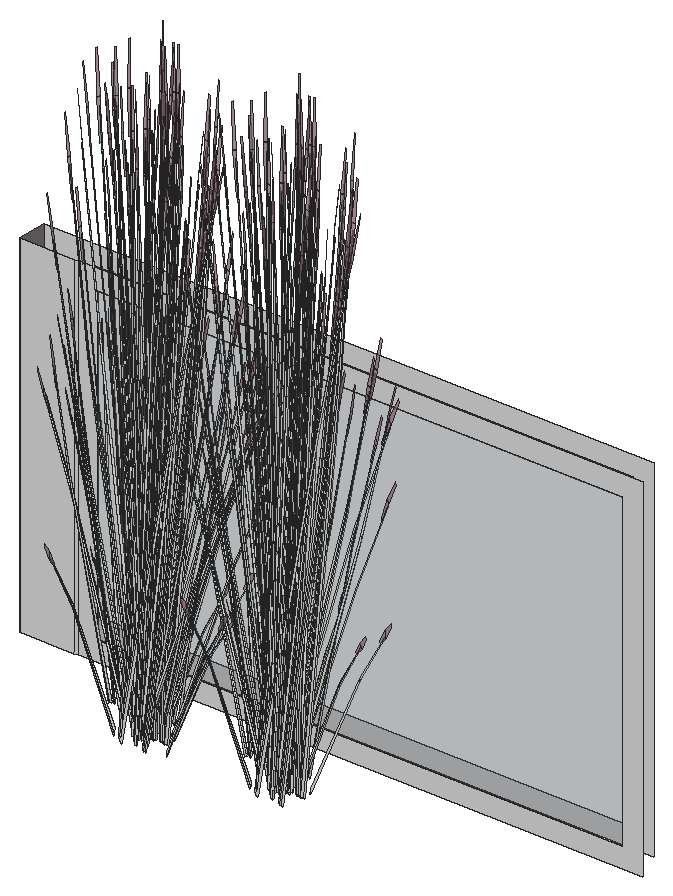
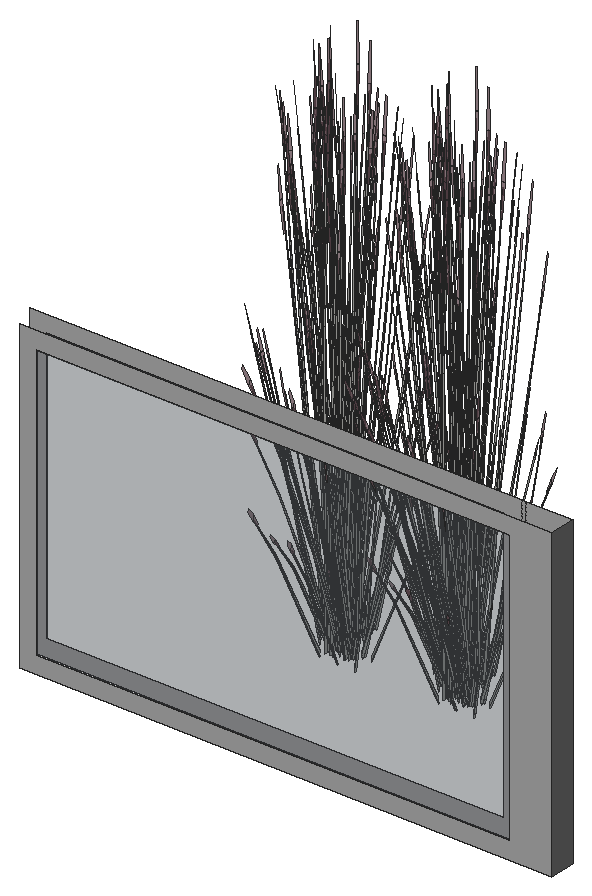
# SketchUp Ruby script. Lengths in inches.
U = 1.inch
M = Sketchup.active_model
def pt(a) = Geom::Point3d.new(a.map { |v| v * U })
def face(e, loops, mat)
  f = e.add_face(loops[0].map { |a| pt(a) })
  loops[1..].each { |l| e.add_face(l.map { |a| pt(a) }).erase! }
  f.material = f.back_material = mat if mat
  f
end
# faces: each face lists its corners as indices into pts; further lists are holes
def faces(e, pts, list, mat = nil) = list.each { |f| face(e, (f[0].is_a?(Array) ? f : [f]).map { |l| l.map { |i| pts[i] } }, mat) }
# xy, xz, yz: faces in a plane at the given z, y or x. An outline is a flat list of corners, or four numbers for a rectangle; further outlines are holes
def ring(l) = l.size == 4 ? [[l[0], l[1]], [l[2], l[1]], [l[2], l[3]], [l[0], l[3]]] : l.each_slice(2).to_a
def flat(e, list, mat, &to3) = list.each { |f| face(e, (f[0].is_a?(Array) ? f : [f]).map { |l| ring(l).map { |u, v| to3.(u, v) } }, mat) }
def xy(e, z, list, mat = nil) = flat(e, list, mat) { |x, y| [x, y, z] }
def xz(e, y, list, mat = nil) = flat(e, list, mat) { |x, z| [x, y, z] }
def yz(e, x, list, mat = nil) = flat(e, list, mat) { |y, z| [x, y, z] }
def lines(e, pts, list) = list.each { |a, b| e.add_line(pt(pts[a]), pt(pts[b])) }
# prism: a flat outline (further loops are holes) pulled along v
def prism(e, loops, v, mat = nil)
  f = face(e, loops, mat); d = Geom::Vector3d.new(v.map { |x| x * U })
  f.pushpull(f.normal.samedirection?(d) ? d.length : -d.length)
end
def box(e, o, s, mat = nil) = prism(e, [[o, [o[0] + s[0], o[1], o[2]], [o[0] + s[0], o[1] + s[1], o[2]], [o[0], o[1] + s[1], o[2]]]], [0, 0, s[2]], mat)
def at(x, y, z, deg = 0) = Geom::Transformation.translation(pt([x, y, z])) * Geom::Transformation.rotation(ORIGIN, Z_AXIS, deg.degrees)
def axes(o, x, y, z) = Geom::Transformation.new([*x, 0, *y, 0, *z, 0, *pt(o).to_a, 1])
def part(name) = M.definitions.add(name)
# library, detail: a bought-in or finely detailed component or shape, given as its bounding box
def library(name, o, s) = part(name).tap { |d| box(d.entities, o, s) }
def detail(e, o, s) = box(e.add_group.entities, o, s)
def put(e, d, t, mat = nil) = e.add_instance(d, t).tap { |i| i.material = mat if mat }
def group(e, t, mat = nil) = e.add_group.tap { |g| g.transformation = t; g.material = mat if mat }.entities
root = M.entities
M.materials.add("Glass_Basic_01").color = [105, 113, 122]
M.materials["Glass_Basic_01"].alpha = 0.25
M.materials.add("LightPink_Translucent").color = [144, 107, 117]
M.materials["LightPink_Translucent"].alpha = 0.75
M.materials.add("M01_Silver_Fog").color = [224, 224, 224]
M.materials.add("M06_Steel_Smoke").color = [114, 114, 114]
c1 = part("blade")
p = [[2.15,0.21,22],[0,0.17,0],[0.09,0.45,0],[2.18,0.31,22],[2.29,0.31,22],[0.38,0.45,0],
  [2.48,0.24,33],[2.49,0.24,33],[2.48,0.22,33]]
faces(c1.entities,p,[[0,1,2,3],[4,5,2,3],[6,3,4,7],[8,0,3,6]])
c2 = part("seeds")
p = [[0.3,-0.1,1.38],[-0.01,-0.03,1.59],[-0.01,-0.03,0.03],[0.14,-0.07,-0.07],[0.29,-0.03,3],[0.15,0.01,3.11]]
faces(c2.entities,p,[[0,1,2,3],[1,0,4,5]],"LightPink_Translucent")
c3 = part("blade with seeds")
put(c3.entities,c1,at(0,0,0))
put(c3.entities,c2,axes([2.4,0.25,30.99],[1.5799,-0.05474,1.17369],[-0.12525,1.92788,0.29478],[-0.07173,-0.02425,1.56792]))
xz(root,474,[[218,650,271.49,682]],"Glass_Basic_01")
xz(root,474,[[210,648,215.53,684],[215.53,648,216,684],[[216,648,273.49,684],[218,650,271.49,682]]],"M01_Silver_Fog")
xz(root,477,[[215,650,270.25,682]],"Glass_Basic_01")
xz(root,477,[[[210,648,272.25,684],[215,650,270.25,682]]],"M01_Silver_Fog")
yz(root,210,[[474,648,477,684]],"M06_Steel_Smoke")
put(root,c3,axes([230.43,461,653.875],[0.17434,-0.11391,1.71376],[0.14677,0.52637,0.13857],[-0.27369,0.11897,0.73262]))
put(root,c3,axes([229.89,461.89,652.59],[0.17462,0.04421,1.43002],[0.11254,0.45156,-0.30754],[-0.23719,0.08453,0.61141]))
put(root,c3,axes([231.43,460.45,653.34],[0.14282,-0.0779,1.77064],[0.04925,0.54394,0.13857],[-0.30935,0.07218,0.63284]))
put(root,c3,axes([230.16,460.52,654.53],[-0.41757,-0.15024,-0.35414],[0.12179,-0.4383,0.4572],[-0.16812,0.04019,0.87481]))
put(root,c3,axes([230.44,460.74,654.68],[-0.13612,0.48987,-0.51099],[-0.46669,-0.16791,-0.3958],[-0.1879,0.04492,0.97773]))
put(root,c3,axes([230.21,460.71,651.49],[0.01274,0.08487,1.76342],[-0.25688,0.44323,-0.26939],[-0.18246,-0.02234,0.30037]))
put(root,c3,axes([229.52,462.84,652.77],[0.2094,-0.24408,1.1486],[0.08263,0.38639,0.84392],[-0.15132,0.06919,0.25299]))
put(root,c3,axes([231.07,461.35,653.875],[0.1255,-0.16547,1.71376],[0.31687,0.44665,0.13857],[-0.21734,0.2034,0.73262]))
put(root,c3,axes([230.3125,461.78,654.53],[-0.43736,0.07697,-0.35414],[-0.11549,-0.43998,0.4572],[-0.12533,0.11818,0.87481]))
put(root,c3,axes([230.07,463.09,651.49],[0.0674,0.0538,1.76342],[0.11428,0.49852,-0.26939],[-0.14937,0.10631,0.30037]))
put(root,c3,axes([230.97,461.76,653.875],[0.09355,-0.18511,1.71376],[0.39247,0.38307,0.13857],[-0.17705,0.23875,0.73262]))
put(root,c3,axes([230.67,461.83,654.68],[0.12908,0.49174,-0.51099],[-0.48882,0.08602,-0.3958],[-0.14008,0.13208,0.97773]))
put(root,c3,axes([231.89,461.48,652.06],[-0.52267,-0.08829,-0.62353],[0.11029,-0.54463,-0.16365],[-0.15598,-0.06599,1.37633]))
put(root,c3,axes([231.2,462.51,652.02],[-0.47024,-0.26927,-0.49651],[0.28107,-0.48284,0],[-0.1071,-0.06133,1.57504]))
put(root,c3,axes([231.49,462.84,652.375],[-0.31414,0.53965,0],[-0.52557,-0.30095,-0.51607],[-0.1197,-0.06854,1.63711]))
put(root,c3,axes([230.92,463.62,652.59],[0.15856,-0.08496,1.43002],[0.39147,0.25616,-0.30754],[-0.11652,0.22165,0.61141]))
put(root,c3,axes([232.48,461.5625,652.67],[-0.5073,0.35754,-0.29095],[-0.33735,-0.5052,-0.50002],[-0.12516,-0.05131,1.59708]))
put(root,c3,axes([231.34,462.3125,652.03],[-0.11803,-0.46926,-0.30978],[0.46876,-0.13325,0.30978],[-0.0945,-0.05411,1.38974]))
put(root,c3,axes([231.08,462.8,654.53],[-0.33997,0.28354,-0.35414],[-0.32182,-0.32376,0.4572],[-0.04897,0.1645,0.87481]))
put(root,c3,axes([232.82,461.95,652.06],[-0.33843,0.40479,-0.62353],[-0.42041,-0.36705,-0.16365],[-0.13561,0.10098,1.37633]))
put(root,c3,axes([233.05,461.73,652.46],[-0.49063,-0.43346,-0.25192],[0.41285,-0.48673,0.5513],[-0.13212,0.05071,1.68216]))
put(root,c3,axes([231.31,462.5,655.34],[-0.01307,0.49815,-0.7886],[-0.55054,-0.03346,0.09517],[-0.0581,0.21104,1.11556]))
put(root,c3,axes([231.3,463.9,652.77],[-0.013,-0.32022,1.1486],[0.32493,0.22839,0.84392],[-0.0639,0.15263,0.25299]))
put(root,c3,axes([232.8,461.63,652.21],[-0.54562,0.03324,-0.44739],[-0.04934,-0.55185,0.21531],[-0.09768,0.05593,1.43643]))
put(root,c3,axes([231.76,462.56,652.48],[0.47024,0.26927,0.49651],[-0.28107,0.48284,0],[-0.1071,-0.06133,1.57504]))
put(root,c3,axes([231.12,463.2,653.36],[0.01104,-0.27801,1.54345],[0.49652,0.14685,0.21329],[-0.04302,0.2963,0.72882]))
put(root,c3,axes([232.44,461.72,652.62],[-0.09693,0.48062,0.1448],[-0.47357,-0.08343,-0.41347],[-0.08619,-0.04935,1.26744]))
put(root,c3,axes([233.38,463.06,652.02],[-0.47024,0.26927,-0.49651],[-0.28107,-0.48284,0],[-0.1071,0.06133,1.57504]))
put(root,c3,axes([233.41,462.91,652.19],[-0.31023,-0.54153,-0.05142],[0.52557,-0.30095,0.51607],[-0.12951,0.05156,1.6363]))
put(root,c3,axes([231.42,462.67,655],[0.35968,0.36185,-0.5672],[-0.37996,0.3169,-0.43934],[-0.05473,0.18385,1.08528]))
put(root,c3,axes([233.27,462.84,652.03],[-0.46876,-0.13325,-0.30978],[0.11803,-0.46926,0.30978],[-0.0945,0.05411,1.38974]))
put(root,c3,axes([233.54,460.84,652.84],[-0.01373,-0.50706,1.41272],[0.62119,0.13144,0.59816],[-0.14692,0.27746,1.3335]))
put(root,c3,axes([231.03,463.21,652.82],[0.45645,-0.09537,0.06507],[0.10494,0.38421,-0.86304],[-0.02894,0.19449,0.7736]))
put(root,c3,axes([233.1875,461.48,652.67],[0.05855,0.61451,-0.29095],[-0.60981,0.03716,-0.50002],[-0.10738,0.08185,1.59708]))
put(root,c3,axes([231.83,462.15,653.875],[-0.0123,-0.2067,1.71376],[0.53301,0.13712,0.13857],[-0.03297,0.29456,0.73262]))
put(root,c3,axes([232.28,461.26,652.36],[0.63506,0.11347,0.45755],[-0.12924,0.64083,0.17955],[-0.09281,-0.06188,1.58856]))
put(root,c3,axes([232.11,461.14,652.72],[-0.24378,0.48527,0.44739],[-0.50654,-0.23354,-0.21531],[0,-0.11186,1.43643]))
put(root,c3,axes([231.9375,462.28,652.47],[0.53992,-0.14294,0.17642],[0.13332,0.53195,0.35086],[-0.04815,-0.07751,1.60407]))
put(root,c3,axes([232.63,462.37,652.2],[-0.50654,-0.24178,0],[0.24378,-0.50239,0],[0,0,1.62707]))
put(root,c3,axes([233.8,462.97,652.375],[0.31414,0.53965,0],[-0.52557,0.30095,-0.51607],[-0.1197,0.06854,1.63711]))
put(root,c3,axes([233.54,462.3125,652.47],[0.14515,-0.53522,0.17642],[0.53115,0.15146,0.35086],[-0.09175,0.00261,1.60407]))
put(root,c3,axes([233.3,461.6,652.62],[0.37121,0.32357,0.1448],[-0.30963,0.36505,-0.41347],[-0.08619,0.04935,1.26744]))
put(root,c3,axes([233.17,461.2,652.3],[-0.46736,-0.46353,-0.06131],[0.46764,-0.46381,0],[-0.01632,-0.01619,1.75571]))
put(root,c3,axes([233.29,461.37,652.72],[0.54562,-0.03324,0.44739],[0.04934,0.55185,-0.21531],[-0.09768,0.05593,1.43643]))
put(root,c3,axes([233.42,462.63,652.33],[0.62903,0.17504,0.30756],[-0.15737,0.62568,-0.36492],[-0.10411,0.07831,1.64885]))
put(root,c3,axes([233.69,462.6,652.48],[0.47024,-0.26927,0.49651],[0.28107,0.48284,0],[-0.1071,0.06133,1.57504]))
put(root,c3,axes([232.75,462.16,652.2],[-0.16394,-0.4643,0],[0.46814,-0.1626,0],[0,0,1.54371]))
put(root,c3,axes([232.15,463.14,651.49],[0.08132,-0.0293,1.76342],[0.48914,0.1613,-0.26939],[0.0143,0.18179,0.30037]))
put(root,c3,axes([232.26,463.3,654.53],[-0.15148,0.41415,-0.35414],[-0.44193,-0.12079,0.4572],[0.04052,0.16674,0.87481]))
put(root,c3,axes([233.41,461.24,652.21],[-0.24378,0.48527,-0.44739],[-0.50654,-0.23354,0.21531],[0,0.11186,1.43643]))
put(root,c3,axes([234.375,460.95,652.47],[-0.39477,-0.39228,0.17642],[0.39783,-0.38049,0.35086],[-0.0436,0.08011,1.60407]))
put(root,c3,axes([233.01,460.72,652.21],[0,-0.62313,0],[0.62828,0,0],[0,0,1.79456]))
put(root,c3,axes([233.33,460.97,652.29],[0,0.62282,-0.05637],[-0.62828,0,0],[0,0.01957,1.79368]))
put(root,c3,axes([231.99,459.52,652.47],[-0.14515,0.53522,0.17642],[-0.53115,-0.15146,0.35086],[0.09175,-0.00261,1.60407]))
put(root,c3,axes([233.03,462.18,652.29],[0.21845,0.61869,-0.06012],[-0.62418,0.21679,0],[0.00763,0.02161,1.72173]))
put(root,c3,axes([232.31,462.93,654.98],[0.23981,0.43789,-0.71045],[-0.49365,0.24404,0.08574],[0.05608,0.21158,1.00501]))
put(root,c3,axes([234.83,461.36,652.2],[-0.62797,-0.00431,-0.04976],[0,-0.6019,0.49943],[-0.01973,0.13702,1.58352]))
put(root,c3,axes([233.6,459.55,652.47],[-0.53992,0.14294,0.17642],[-0.13332,-0.53195,0.35086],[0.04815,0.07751,1.60407]))
put(root,c3,axes([232.71,460.33,652.36],[-0.4166,0.48873,0.45755],[-0.49494,-0.43142,0.17955],[0.10044,-0.04877,1.58856]))
put(root,c3,axes([233.42,461.1,652.21],[0.35073,0.34786,0],[-0.35073,0.34786,0],[0,0,1.69266]))
put(root,c3,axes([233.42,460.69,652.72],[0.24378,-0.48527,0.44739],[0.50654,0.23354,-0.21531],[0,0.11186,1.43643]))
put(root,c3,axes([233.21,462.38,652.2],[0.50654,0.24178,0],[-0.24378,0.50239,0],[0,0,1.74954]))
put(root,c3,axes([232.49,463.02,654.68],[0.49392,0.135,-0.51099],[-0.1693,0.46287,-0.3958],[0.04529,0.18636,0.97773]))
put(root,c3,axes([233.25,460.58,652.38],[-0.63506,-0.11347,0.49198],[0.12924,-0.64083,0.19306],[0.09281,0.06188,1.70813]))
put(root,c3,axes([234.7,461.45,652.03],[-0.35073,0.33601,-0.30978],[-0.35073,-0.33601,0.30978],[0,0.10823,1.38974]))
put(root,c3,axes([233.7,461.39,652.09],[0.18424,0.49308,-0.69212],[-0.53071,0.17758,-0.18165],[0.02036,0.16697,1.52773]))
put(root,c3,axes([233.4375,460.86,652.21],[0.56215,0,0],[0,0.55754,0],[0,0,1.78407]))
put(root,c3,axes([232.9,460.25,652.72],[-0.30184,-0.45202,0.44739],[0.45719,-0.31831,-0.21531],[0.09768,0.05593,1.43643]))
put(root,c3,axes([233.63,460.8,652.62],[0.46814,-0.15705,0.1448],[0.16394,0.44848,-0.41347],[0,0.0987,1.26744]))
put(root,c3,axes([233.47,460.84,652.67],[0.56585,0.25696,-0.29095],[-0.27246,0.54236,-0.50002],[0.01778,0.13316,1.59708]))
put(root,c3,axes([234.7,460.96,652.48],[0,-0.53854,0.49651],[0.56215,0,0],[0,0.12266,1.57504]))
put(root,c3,axes([234.94,461.46,652.02],[0,0.53854,-0.49651],[-0.56215,0,0],[0,0.12266,1.57504]))
put(root,c3,axes([232.77,462.0625,653.875],[-0.11485,-0.17291,1.71376],[0.53072,-0.14557,0.13857],[0.11995,0.27145,0.73262]))
put(root,c3,axes([233.1,460.12,652.62],[0.09693,-0.48062,0.1448],[0.47357,0.08343,-0.41347],[0.08619,0.04935,1.26744]))
put(root,c3,axes([233.77,459.28,652.48],[-0.47024,-0.26927,0.49651],[0.28107,-0.48284,0],[0.1071,0.06133,1.57504]))
put(root,c3,axes([233.36,462.09,652.18],[0.5275,-0.18273,-0.19198],[0.18536,0.52636,0.00008],[0.05823,-0.0202,1.73897]))
put(root,c3,axes([233.37,460.53,652.21],[0.30184,0.45202,-0.44739],[-0.45719,0.31831,0.21531],[0.09768,0.05593,1.43643]))
put(root,c3,axes([234.23,462.58,652.77],[-0.2829,-0.15485,1.1486],[0.36529,-0.15734,0.84392],[0.09853,0.13328,0.25299]))
put(root,c3,axes([233.22,462.41,652.59],[0.00887,-0.17852,1.43002],[0.42372,-0.19941,-0.30754],[0.1308,0.21367,0.61141]))
put(root,c3,axes([234.2,459.53,652.03],[0.11803,0.46926,-0.30978],[-0.46876,0.13325,0.30978],[0.0945,0.05411,1.38974]))
put(root,c3,axes([235.08,461.05,652.375],[0.62828,0,0],[0,0.6019,-0.51607],[0,0.13709,1.63711]))
put(root,c3,axes([233.05,460.27,652.67],[0.5073,-0.35754,-0.29095],[0.33735,0.5052,-0.50002],[0.12516,0.05131,1.59708]))
put(root,c3,axes([234.27,463.28,652.67],[-0.3222,-0.01689,1.0506],[0.21278,-0.35872,0.58006],[0.12729,0.12745,0.8241]))
put(root,c3,axes([231.77,459.96,651.59],[-0.49456,0.21561,1.28929],[-0.15741,-0.61865,0.50096],[0.30369,0.01029,1.46642]))
put(root,c3,axes([233.59,462.79,654.68],[0.4958,-0.12802,-0.51099],[0.08673,0.48481,-0.3958],[0.13317,0.13893,0.97773]))
put(root,c3,axes([234.33,459.32,652.02],[0.47024,0.26927,-0.49651],[-0.28107,0.48284,0],[0.1071,0.06133,1.57504]))
put(root,c3,axes([234.31,463.16,651.49],[0.03661,-0.07775,1.76342],[0.46087,-0.22898,-0.26939],[0.13972,0.11851,0.30037]))
put(root,c3,axes([235.41,462.4375,653.93],[-0.09617,-0.45271,-0.03492],[0.45453,-0.10408,-0.15832],[0.09492,0.0287,0.52218]))
put(root,c3,axes([233.64,460.36,652.06],[0.52267,0.08829,-0.62353],[-0.11029,0.54463,-0.16365],[0.15598,0.06599,1.37633]))
put(root,c3,axes([233.53,461.52,653.875],[-0.18664,-0.09279,1.71376],[0.38624,-0.38925,0.13857],[0.24072,0.1756,0.73262]))
put(root,c3,axes([234.5625,462.39,654.53],[0.28589,0.33718,-0.35414],[-0.32644,0.31919,0.4572],[0.16586,0.04856,0.87481]))
put(root,c3,axes([235.95,461.31,652.77],[-0.31044,0.08891,1.1486],[0.14613,-0.36744,0.84392],[0.16469,0.02514,0.25299]))
put(root,c3,axes([235.07,461.22,654.53],[0.41757,0.15024,-0.35414],[-0.12179,0.4383,0.4572],[0.16812,-0.04019,0.87481]))
put(root,c3,axes([234.26,462.16,654.98],[0.50227,0.01297,-0.71045],[-0.03373,0.54602,0.08574],[0.21278,0.05762,1.00501]))
put(root,c3,axes([235.63,460.8,651.49],[-0.02626,-0.08176,1.76342],[0.18213,-0.47826,-0.26939],[0.18372,-0.00688,0.30037]))
put(root,c3,axes([233.93,460.67,653.875],[-0.20841,0.0122,1.71376],[0.13825,-0.52864,0.13857],[0.297,0.0327,0.73262]))
put(root,c3,axes([234.69,461.17,654.98],[0.44151,-0.23785,-0.71045],[0.24605,0.4896,0.08574],[0.21333,-0.05562,1.00501]))
put(root,c3,axes([244.32,461,653.875],[0.17434,-0.11391,1.71376],[0.14677,0.52637,0.13857],[-0.27369,0.11897,0.73262]))
put(root,c3,axes([235.37,461.9,652.59],[-0.12101,-0.13245,1.43002],[0.15744,-0.43816,-0.30754],[0.24483,0.05936,0.61141]))
put(root,c3,axes([243.77,461.89,652.59],[0.17462,0.04421,1.43002],[0.11254,0.45156,-0.30754],[-0.23719,0.08453,0.61141]))
put(root,c3,axes([245.32,460.45,653.34],[0.14282,-0.0779,1.77064],[0.04925,0.54394,0.13857],[-0.30935,0.07218,0.63284]))
put(root,c3,axes([244.05,460.52,654.53],[-0.41757,-0.15024,-0.35414],[0.12179,-0.4383,0.4572],[-0.16812,0.04019,0.87481]))
put(root,c3,axes([244.33,460.74,654.68],[-0.13612,0.48987,-0.51099],[-0.46669,-0.16791,-0.3958],[-0.1879,0.04492,0.97773]))
put(root,c3,axes([244.1,460.71,651.49],[0.01274,0.08487,1.76342],[-0.25688,0.44323,-0.26939],[-0.18246,-0.02234,0.30037]))
put(root,c3,axes([243.41,462.84,652.77],[0.2094,-0.24408,1.1486],[0.08263,0.38639,0.84392],[-0.15132,0.06919,0.25299]))
put(root,c3,axes([244.95,461.35,653.875],[0.1255,-0.16547,1.71376],[0.31687,0.44665,0.13857],[-0.21734,0.2034,0.73262]))
put(root,c3,axes([244.2,461.78,654.53],[-0.43736,0.07697,-0.35414],[-0.11549,-0.43998,0.4572],[-0.12533,0.11818,0.87481]))
put(root,c3,axes([243.96,463.09,651.49],[0.0674,0.0538,1.76342],[0.11428,0.49852,-0.26939],[-0.14937,0.10631,0.30037]))
put(root,c3,axes([244.86,461.76,653.875],[0.09355,-0.18511,1.71376],[0.39247,0.38307,0.13857],[-0.17705,0.23875,0.73262]))
put(root,c3,axes([244.56,461.83,654.68],[0.12908,0.49174,-0.51099],[-0.48882,0.08602,-0.3958],[-0.14008,0.13208,0.97773]))
put(root,c3,axes([245.78,461.48,652.06],[-0.52267,-0.08829,-0.62353],[0.11029,-0.54463,-0.16365],[-0.15598,-0.06599,1.37633]))
put(root,c3,axes([245.09,462.51,652.02],[-0.47024,-0.26927,-0.49651],[0.28107,-0.48284,0],[-0.1071,-0.06133,1.57504]))
put(root,c3,axes([245.38,462.84,652.375],[-0.31414,0.53965,0],[-0.52557,-0.30095,-0.51607],[-0.1197,-0.06854,1.63711]))
put(root,c3,axes([244.8,463.62,652.59],[0.15856,-0.08496,1.43002],[0.39147,0.25616,-0.30754],[-0.11652,0.22165,0.61141]))
put(root,c3,axes([246.37,461.5625,652.67],[-0.5073,0.35754,-0.29095],[-0.33735,-0.5052,-0.50002],[-0.12516,-0.05131,1.59708]))
put(root,c3,axes([245.22,462.3125,652.03],[-0.11803,-0.46926,-0.30978],[0.46876,-0.13325,0.30978],[-0.0945,-0.05411,1.38974]))
put(root,c3,axes([244.97,462.8,654.53],[-0.33997,0.28354,-0.35414],[-0.32182,-0.32376,0.4572],[-0.04897,0.1645,0.87481]))
put(root,c3,axes([246.71,461.95,652.06],[-0.33843,0.40479,-0.62353],[-0.42041,-0.36705,-0.16365],[-0.13561,0.10098,1.37633]))
put(root,c3,axes([246.94,461.73,652.46],[-0.49063,-0.43346,-0.25192],[0.41285,-0.48673,0.5513],[-0.13212,0.05071,1.68216]))
put(root,c3,axes([245.19,462.5,655.34],[-0.01307,0.49815,-0.7886],[-0.55054,-0.03346,0.09517],[-0.0581,0.21104,1.11556]))
put(root,c3,axes([245.18,463.9,652.77],[-0.013,-0.32022,1.1486],[0.32493,0.22839,0.84392],[-0.0639,0.15263,0.25299]))
put(root,c3,axes([246.69,461.63,652.21],[-0.54562,0.03324,-0.44739],[-0.04934,-0.55185,0.21531],[-0.09768,0.05593,1.43643]))
put(root,c3,axes([245.65,462.56,652.48],[0.47024,0.26927,0.49651],[-0.28107,0.48284,0],[-0.1071,-0.06133,1.57504]))
put(root,c3,axes([245.01,463.2,653.36],[0.01104,-0.27801,1.54345],[0.49652,0.14685,0.21329],[-0.04302,0.2963,0.72882]))
put(root,c3,axes([246.32,461.72,652.62],[-0.09693,0.48062,0.1448],[-0.47357,-0.08343,-0.41347],[-0.08619,-0.04935,1.26744]))
put(root,c3,axes([247.26,463.06,652.02],[-0.47024,0.26927,-0.49651],[-0.28107,-0.48284,0],[-0.1071,0.06133,1.57504]))
put(root,c3,axes([247.3,462.91,652.19],[-0.31023,-0.54153,-0.05142],[0.52557,-0.30095,0.51607],[-0.12951,0.05156,1.6363]))
put(root,c3,axes([245.31,462.67,655],[0.35968,0.36185,-0.5672],[-0.37996,0.3169,-0.43934],[-0.05473,0.18385,1.08528]))
put(root,c3,axes([247.15,462.84,652.03],[-0.46876,-0.13325,-0.30978],[0.11803,-0.46926,0.30978],[-0.0945,0.05411,1.38974]))
put(root,c3,axes([247.42,460.84,652.84],[-0.01373,-0.50706,1.41272],[0.62119,0.13144,0.59816],[-0.14692,0.27746,1.3335]))
put(root,c3,axes([244.92,463.21,652.82],[0.45645,-0.09537,0.06507],[0.10494,0.38421,-0.86304],[-0.02894,0.19449,0.7736]))
put(root,c3,axes([247.07,461.48,652.67],[0.05855,0.61451,-0.29095],[-0.60981,0.03716,-0.50002],[-0.10738,0.08185,1.59708]))
put(root,c3,axes([245.71,462.15,653.875],[-0.0123,-0.2067,1.71376],[0.53301,0.13712,0.13857],[-0.03297,0.29456,0.73262]))
put(root,c3,axes([246.17,461.26,652.36],[0.63506,0.11347,0.45755],[-0.12924,0.64083,0.17955],[-0.09281,-0.06188,1.58856]))
put(root,c3,axes([246,461.14,652.72],[-0.24378,0.48527,0.44739],[-0.50654,-0.23354,-0.21531],[0,-0.11186,1.43643]))
put(root,c3,axes([245.82,462.28,652.47],[0.53992,-0.14294,0.17642],[0.13332,0.53195,0.35086],[-0.04815,-0.07751,1.60407]))
put(root,c3,axes([246.52,462.37,652.2],[-0.50654,-0.24178,0],[0.24378,-0.50239,0],[0,0,1.62707]))
put(root,c3,axes([247.69,462.97,652.375],[0.31414,0.53965,0],[-0.52557,0.30095,-0.51607],[-0.1197,0.06854,1.63711]))
put(root,c3,axes([247.43,462.3125,652.47],[0.14515,-0.53522,0.17642],[0.53115,0.15146,0.35086],[-0.09175,0.00261,1.60407]))
put(root,c3,axes([247.1875,461.6,652.62],[0.37121,0.32357,0.1448],[-0.30963,0.36505,-0.41347],[-0.08619,0.04935,1.26744]))
put(root,c3,axes([247.05,461.2,652.3],[-0.46736,-0.46353,-0.06131],[0.46764,-0.46381,0],[-0.01632,-0.01619,1.75571]))
put(root,c3,axes([247.18,461.37,652.72],[0.54562,-0.03324,0.44739],[0.04934,0.55185,-0.21531],[-0.09768,0.05593,1.43643]))
put(root,c3,axes([247.31,462.63,652.33],[0.62903,0.17504,0.30756],[-0.15737,0.62568,-0.36492],[-0.10411,0.07831,1.64885]))
put(root,c3,axes([247.58,462.6,652.48],[0.47024,-0.26927,0.49651],[0.28107,0.48284,0],[-0.1071,0.06133,1.57504]))
put(root,c3,axes([246.64,462.16,652.2],[-0.16394,-0.4643,0],[0.46814,-0.1626,0],[0,0,1.54371]))
put(root,c3,axes([246.04,463.14,651.49],[0.08132,-0.0293,1.76342],[0.48914,0.1613,-0.26939],[0.0143,0.18179,0.30037]))
put(root,c3,axes([246.15,463.3,654.53],[-0.15148,0.41415,-0.35414],[-0.44193,-0.12079,0.4572],[0.04052,0.16674,0.87481]))
put(root,c3,axes([247.3,461.24,652.21],[-0.24378,0.48527,-0.44739],[-0.50654,-0.23354,0.21531],[0,0.11186,1.43643]))
put(root,c3,axes([248.26,460.95,652.47],[-0.39477,-0.39228,0.17642],[0.39783,-0.38049,0.35086],[-0.0436,0.08011,1.60407]))
put(root,c3,axes([246.9,460.72,652.21],[0,-0.62313,0],[0.62828,0,0],[0,0,1.79456]))
put(root,c3,axes([247.21,460.97,652.29],[0,0.62282,-0.05637],[-0.62828,0,0],[0,0.01957,1.79368]))
put(root,c3,axes([245.875,459.52,652.47],[-0.14515,0.53522,0.17642],[-0.53115,-0.15146,0.35086],[0.09175,-0.00261,1.60407]))
put(root,c3,axes([246.91,462.18,652.29],[0.21845,0.61869,-0.06012],[-0.62418,0.21679,0],[0.00763,0.02161,1.72173]))
put(root,c3,axes([246.19,462.93,654.98],[0.23981,0.43789,-0.71045],[-0.49365,0.24404,0.08574],[0.05608,0.21158,1.00501]))
put(root,c3,axes([248.72,461.36,652.2],[-0.62797,-0.00431,-0.04976],[0,-0.6019,0.49943],[-0.01973,0.13702,1.58352]))
put(root,c3,axes([247.48,459.55,652.47],[-0.53992,0.14294,0.17642],[-0.13332,-0.53195,0.35086],[0.04815,0.07751,1.60407]))
put(root,c3,axes([246.6,460.33,652.36],[-0.4166,0.48873,0.45755],[-0.49494,-0.43142,0.17955],[0.10044,-0.04877,1.58856]))
put(root,c3,axes([247.3125,461.1,652.21],[0.35073,0.34786,0],[-0.35073,0.34786,0],[0,0,1.69266]))
put(root,c3,axes([247.31,460.69,652.72],[0.24378,-0.48527,0.44739],[0.50654,0.23354,-0.21531],[0,0.11186,1.43643]))
put(root,c3,axes([247.09,462.38,652.2],[0.50654,0.24178,0],[-0.24378,0.50239,0],[0,0,1.74954]))
put(root,c3,axes([246.37,463.02,654.68],[0.49392,0.135,-0.51099],[-0.1693,0.46287,-0.3958],[0.04529,0.18636,0.97773]))
put(root,c3,axes([247.14,460.58,652.38],[-0.63506,-0.11347,0.49198],[0.12924,-0.64083,0.19306],[0.09281,0.06188,1.70813]))
put(root,c3,axes([248.59,461.45,652.03],[-0.35073,0.33601,-0.30978],[-0.35073,-0.33601,0.30978],[0,0.10823,1.38974]))
put(root,c3,axes([247.58,461.39,652.09],[0.18424,0.49308,-0.69212],[-0.53071,0.17758,-0.18165],[0.02036,0.16697,1.52773]))
put(root,c3,axes([247.32,460.86,652.21],[0.56215,0,0],[0,0.55754,0],[0,0,1.78407]))
put(root,c3,axes([246.78,460.25,652.72],[-0.30184,-0.45202,0.44739],[0.45719,-0.31831,-0.21531],[0.09768,0.05593,1.43643]))
put(root,c3,axes([247.52,460.8,652.62],[0.46814,-0.15705,0.1448],[0.16394,0.44848,-0.41347],[0,0.0987,1.26744]))
put(root,c3,axes([247.36,460.84,652.67],[0.56585,0.25696,-0.29095],[-0.27246,0.54236,-0.50002],[0.01778,0.13316,1.59708]))
put(root,c3,axes([248.59,460.96,652.48],[0,-0.53854,0.49651],[0.56215,0,0],[0,0.12266,1.57504]))
put(root,c3,axes([248.83,461.46,652.02],[0,0.53854,-0.49651],[-0.56215,0,0],[0,0.12266,1.57504]))
put(root,c3,axes([246.65,462.0625,653.875],[-0.11485,-0.17291,1.71376],[0.53072,-0.14557,0.13857],[0.11995,0.27145,0.73262]))
put(root,c3,axes([246.98,460.12,652.62],[0.09693,-0.48062,0.1448],[0.47357,0.08343,-0.41347],[0.08619,0.04935,1.26744]))
put(root,c3,axes([247.66,459.28,652.48],[-0.47024,-0.26927,0.49651],[0.28107,-0.48284,0],[0.1071,0.06133,1.57504]))
put(root,c3,axes([247.25,462.09,652.18],[0.5275,-0.18273,-0.19198],[0.18536,0.52636,0.00008],[0.05823,-0.0202,1.73897]))
put(root,c3,axes([247.26,460.53,652.21],[0.30184,0.45202,-0.44739],[-0.45719,0.31831,0.21531],[0.09768,0.05593,1.43643]))
put(root,c3,axes([248.11,462.58,652.77],[-0.2829,-0.15485,1.1486],[0.36529,-0.15734,0.84392],[0.09853,0.13328,0.25299]))
put(root,c3,axes([247.11,462.41,652.59],[0.00887,-0.17852,1.43002],[0.42372,-0.19941,-0.30754],[0.1308,0.21367,0.61141]))
put(root,c3,axes([248.08,459.53,652.03],[0.11803,0.46926,-0.30978],[-0.46876,0.13325,0.30978],[0.0945,0.05411,1.38974]))
put(root,c3,axes([248.97,461.05,652.375],[0.62828,0,0],[0,0.6019,-0.51607],[0,0.13709,1.63711]))
put(root,c3,axes([246.9375,460.27,652.67],[0.5073,-0.35754,-0.29095],[0.33735,0.5052,-0.50002],[0.12516,0.05131,1.59708]))
put(root,c3,axes([248.16,463.28,652.67],[-0.3222,-0.01689,1.0506],[0.21278,-0.35872,0.58006],[0.12729,0.12745,0.8241]))
put(root,c3,axes([245.66,459.96,651.59],[-0.49456,0.21561,1.28929],[-0.15741,-0.61865,0.50096],[0.30369,0.01029,1.46642]))
put(root,c3,axes([247.47,462.79,654.68],[0.4958,-0.12802,-0.51099],[0.08673,0.48481,-0.3958],[0.13317,0.13893,0.97773]))
put(root,c3,axes([248.22,459.32,652.02],[0.47024,0.26927,-0.49651],[-0.28107,0.48284,0],[0.1071,0.06133,1.57504]))
put(root,c3,axes([248.19,463.16,651.49],[0.03661,-0.07775,1.76342],[0.46087,-0.22898,-0.26939],[0.13972,0.11851,0.30037]))
